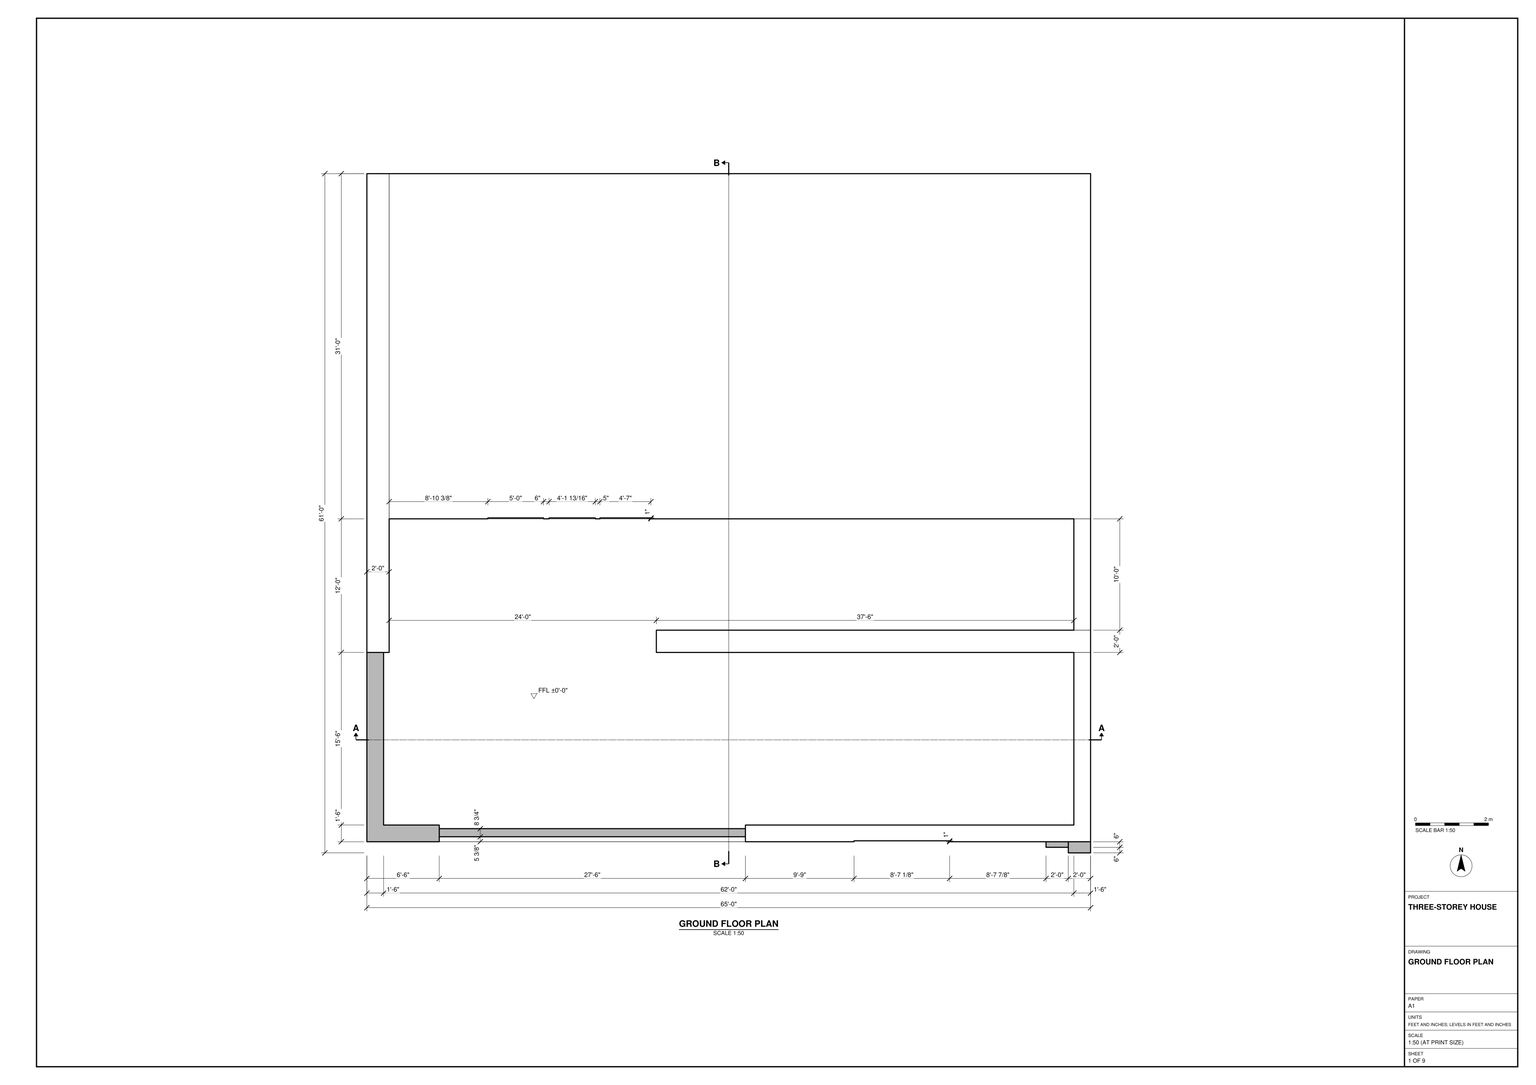
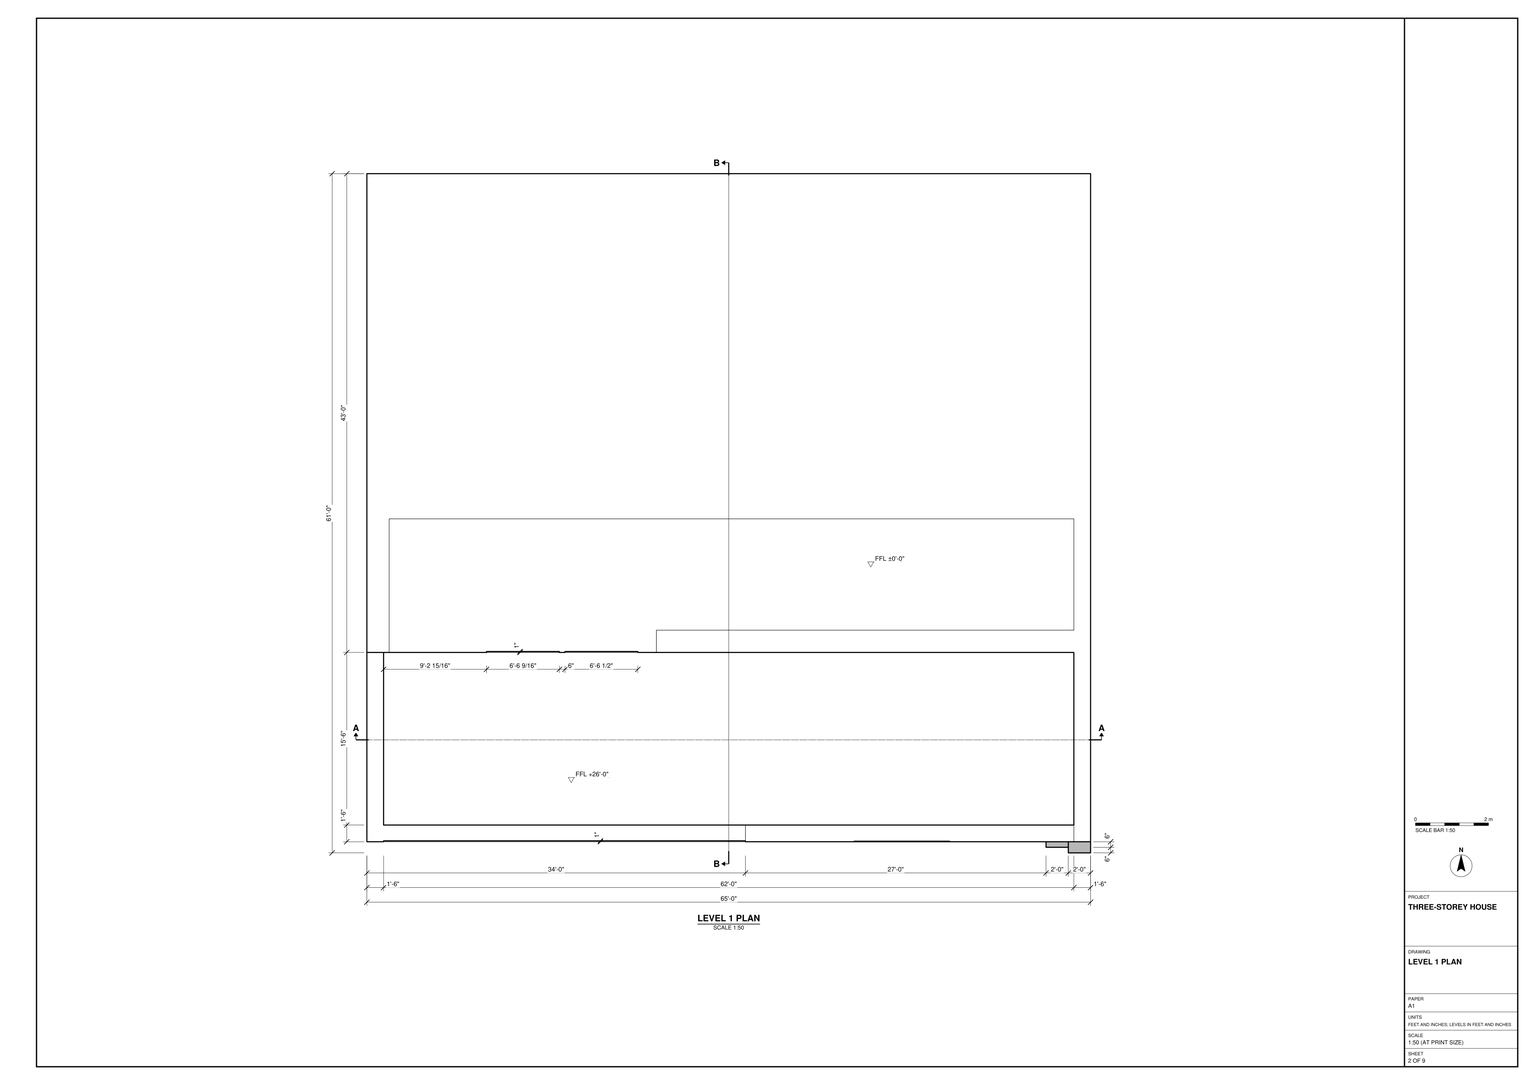
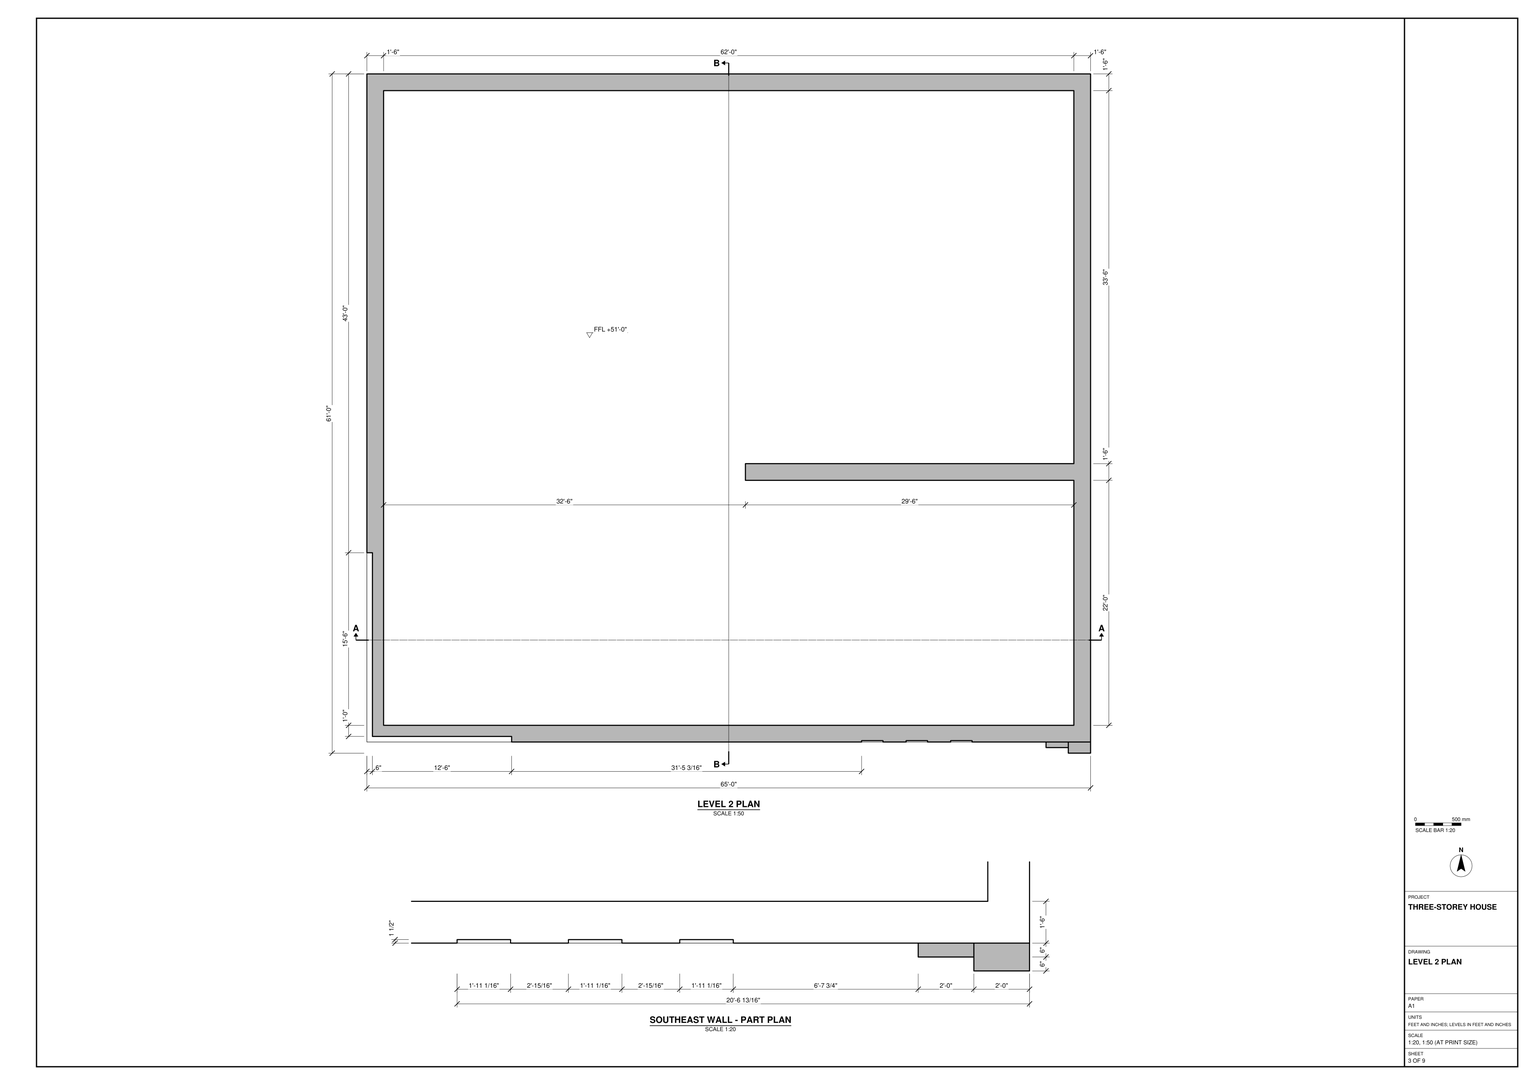
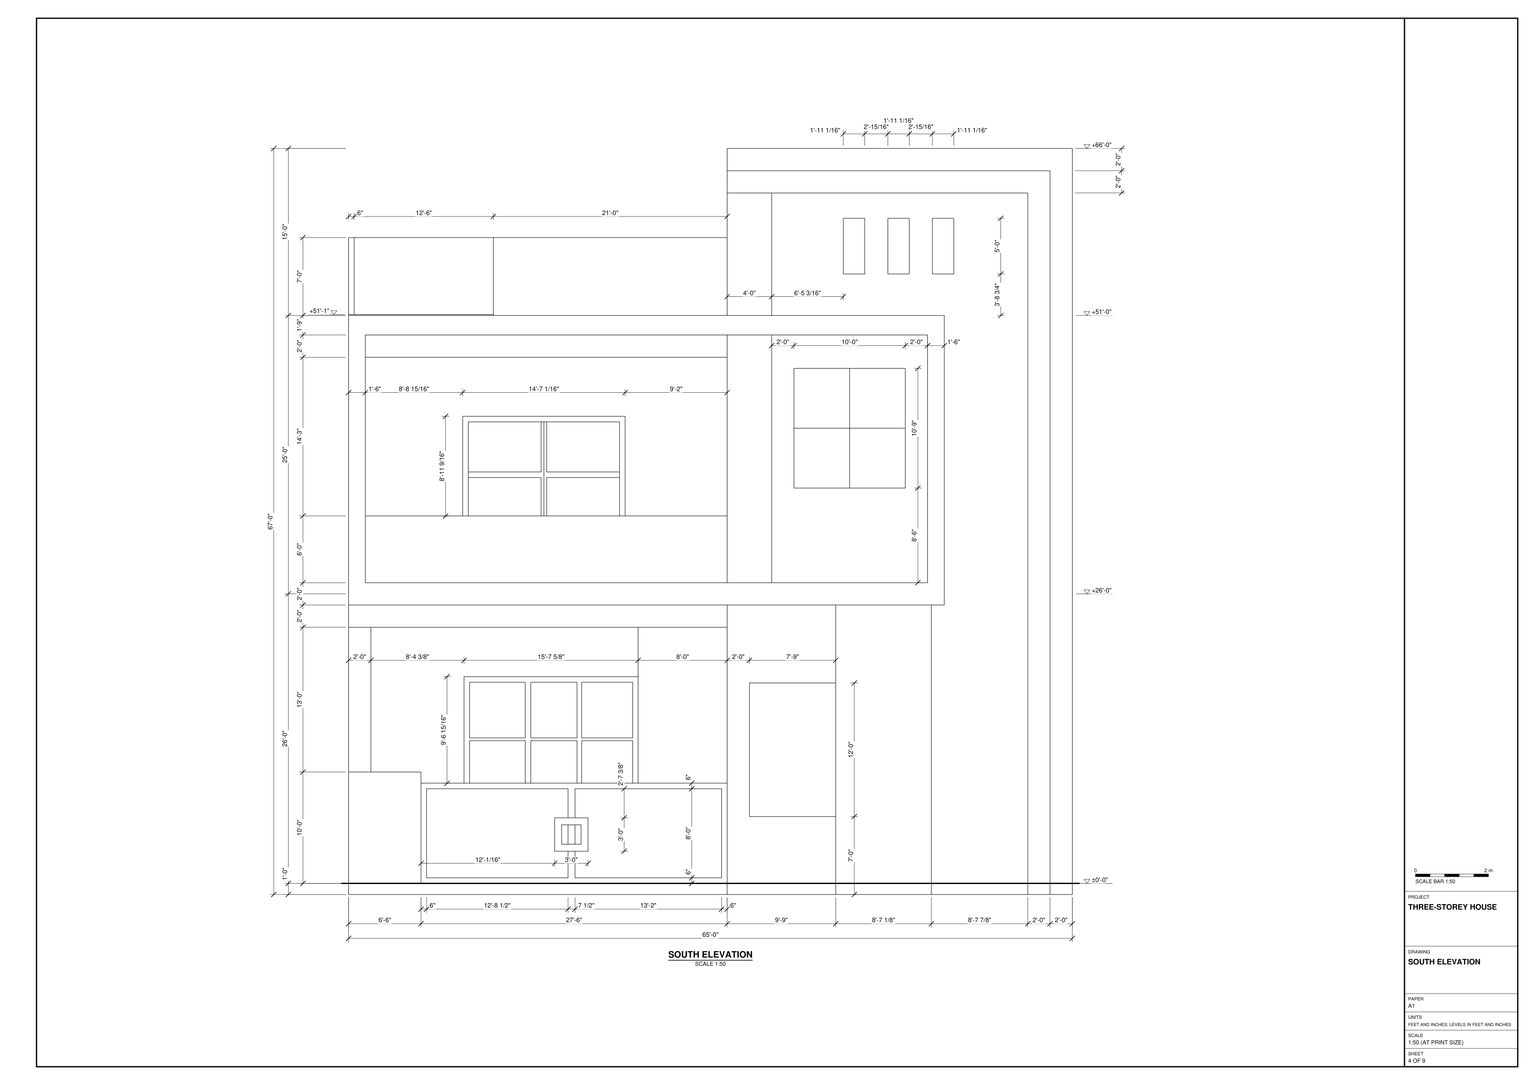
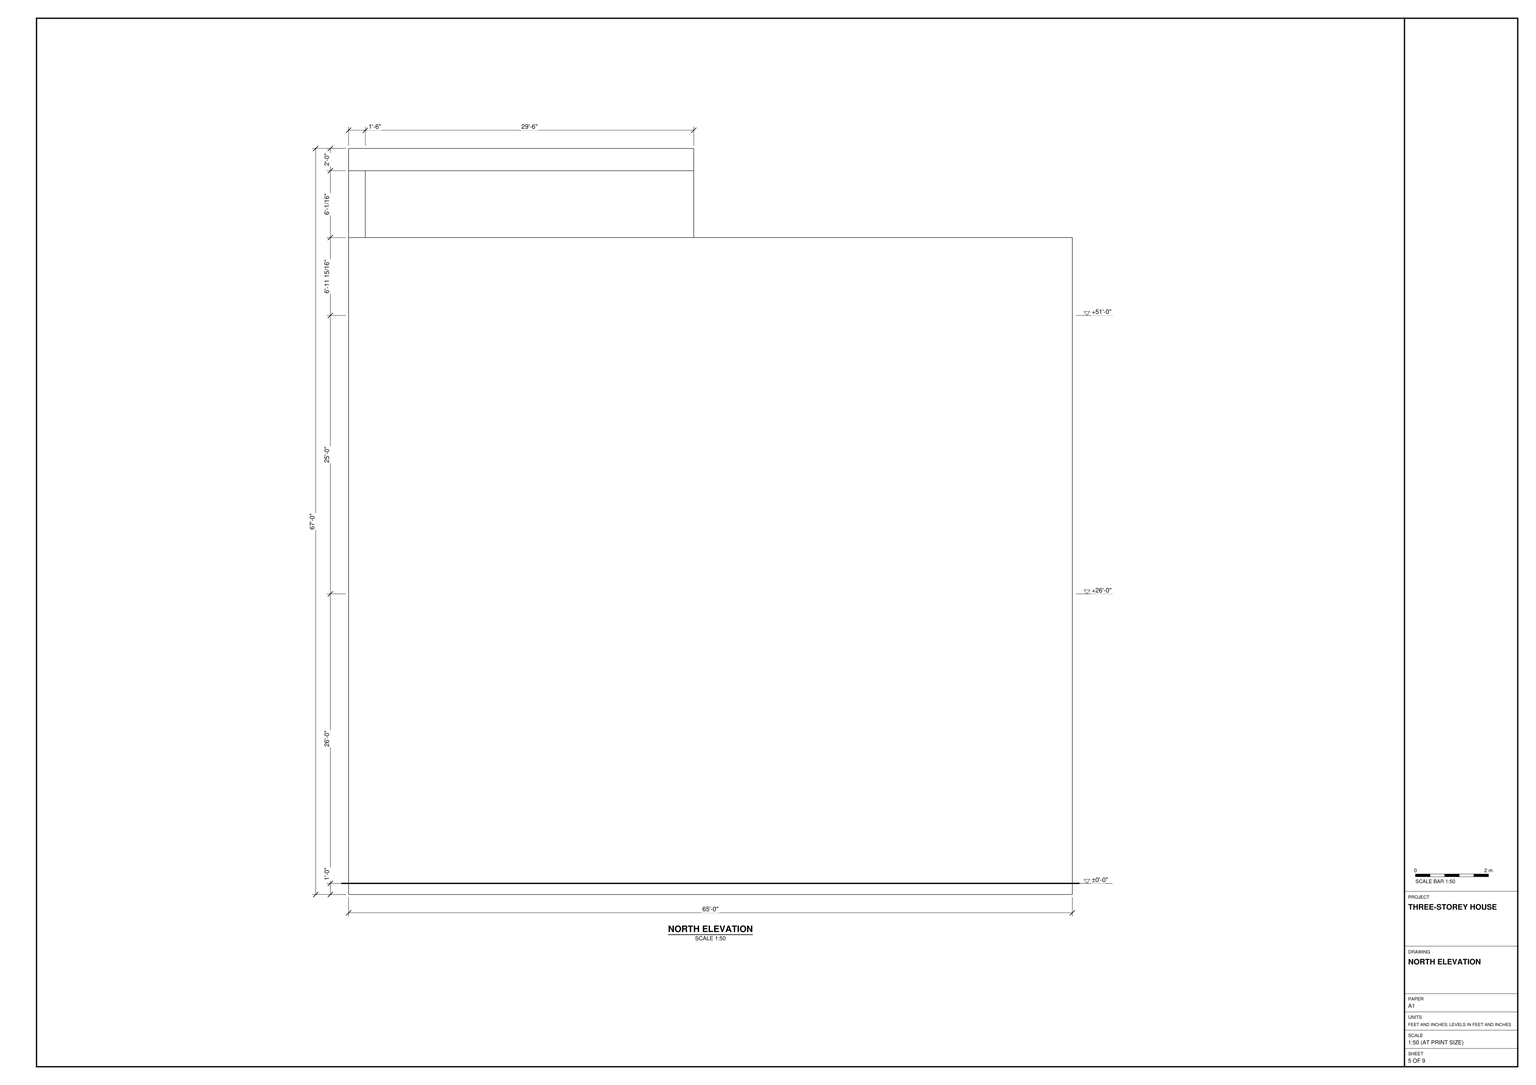
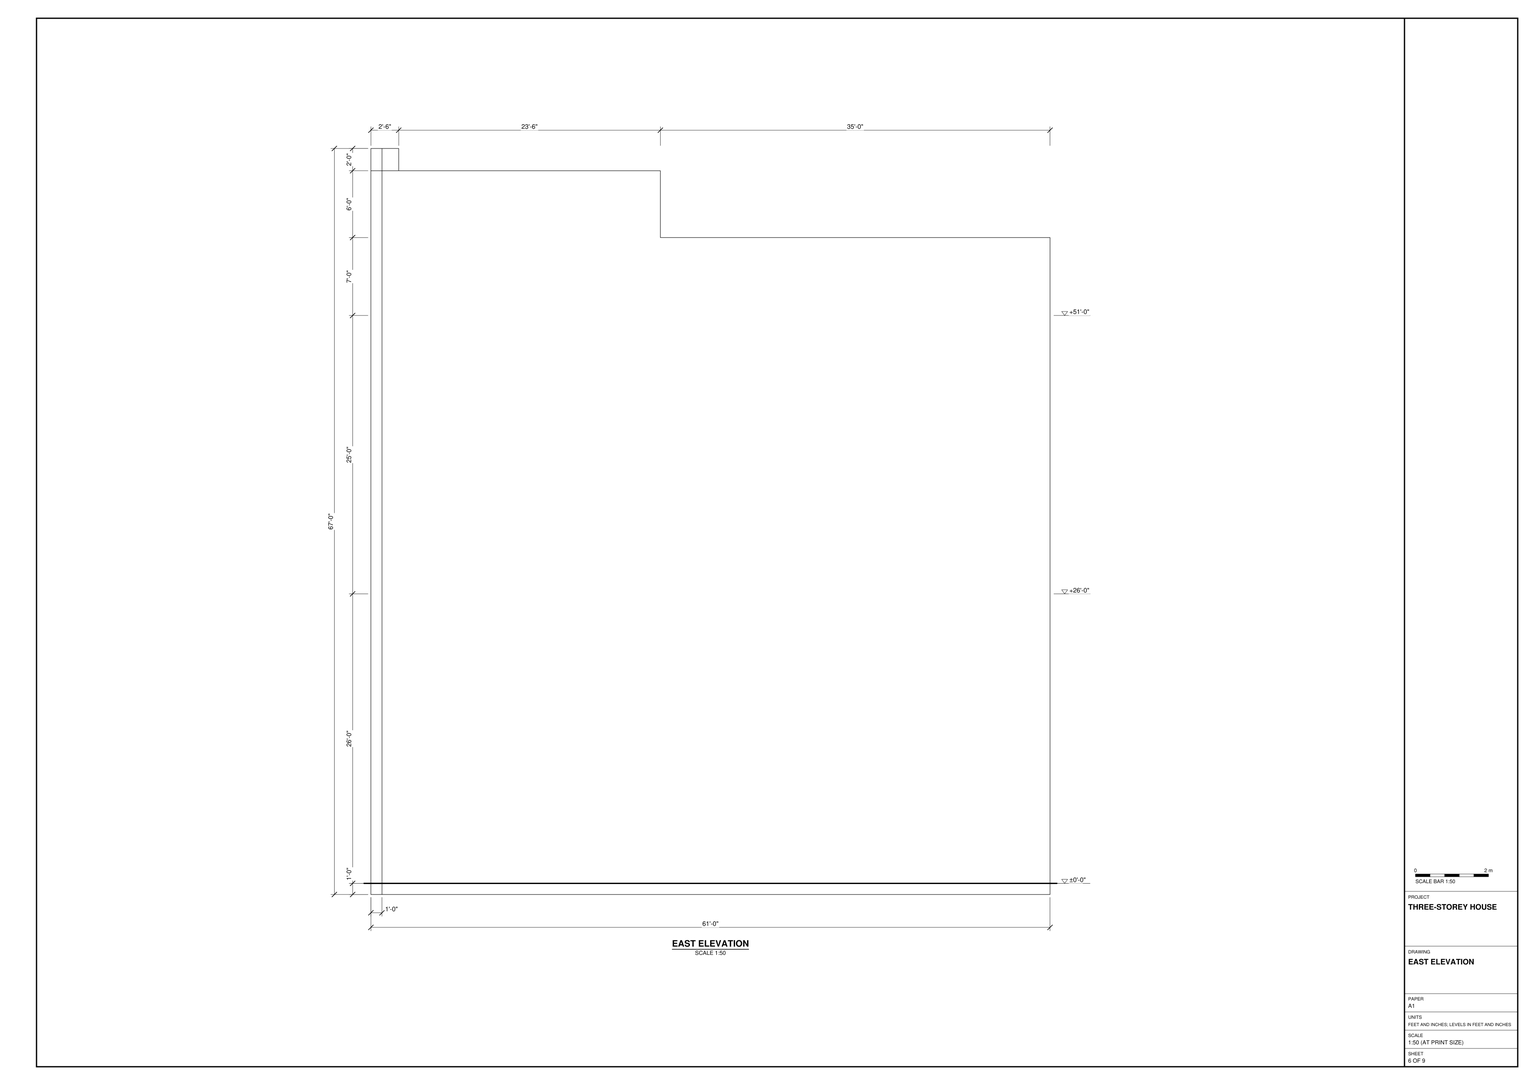
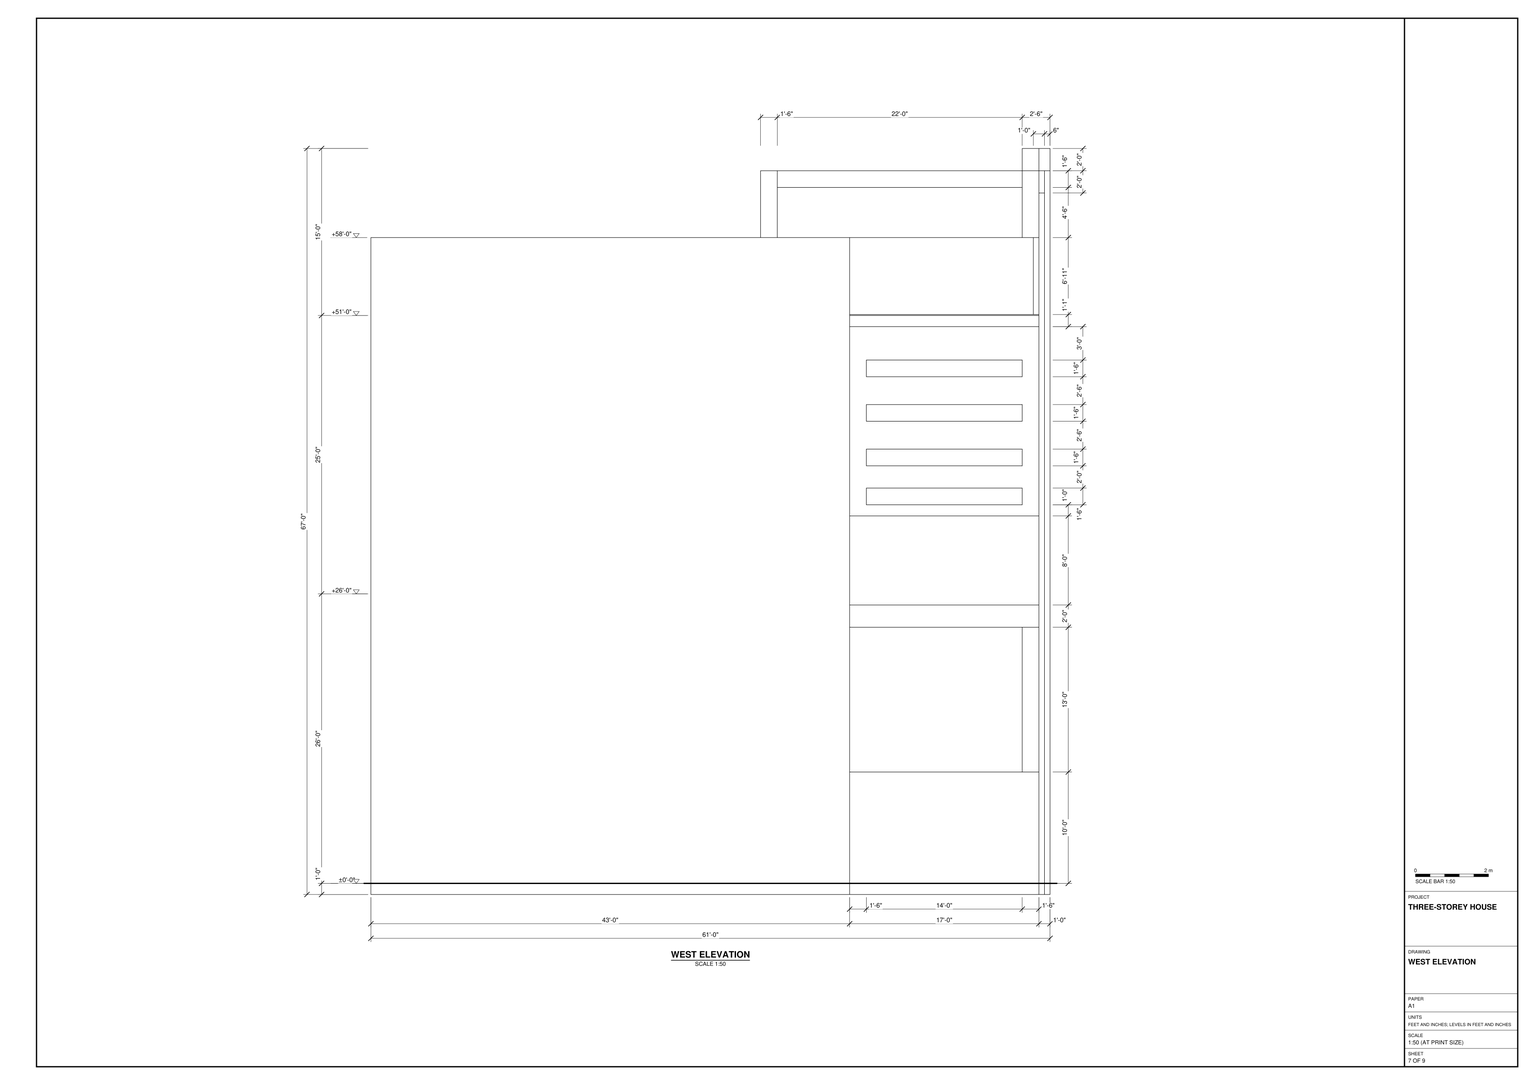
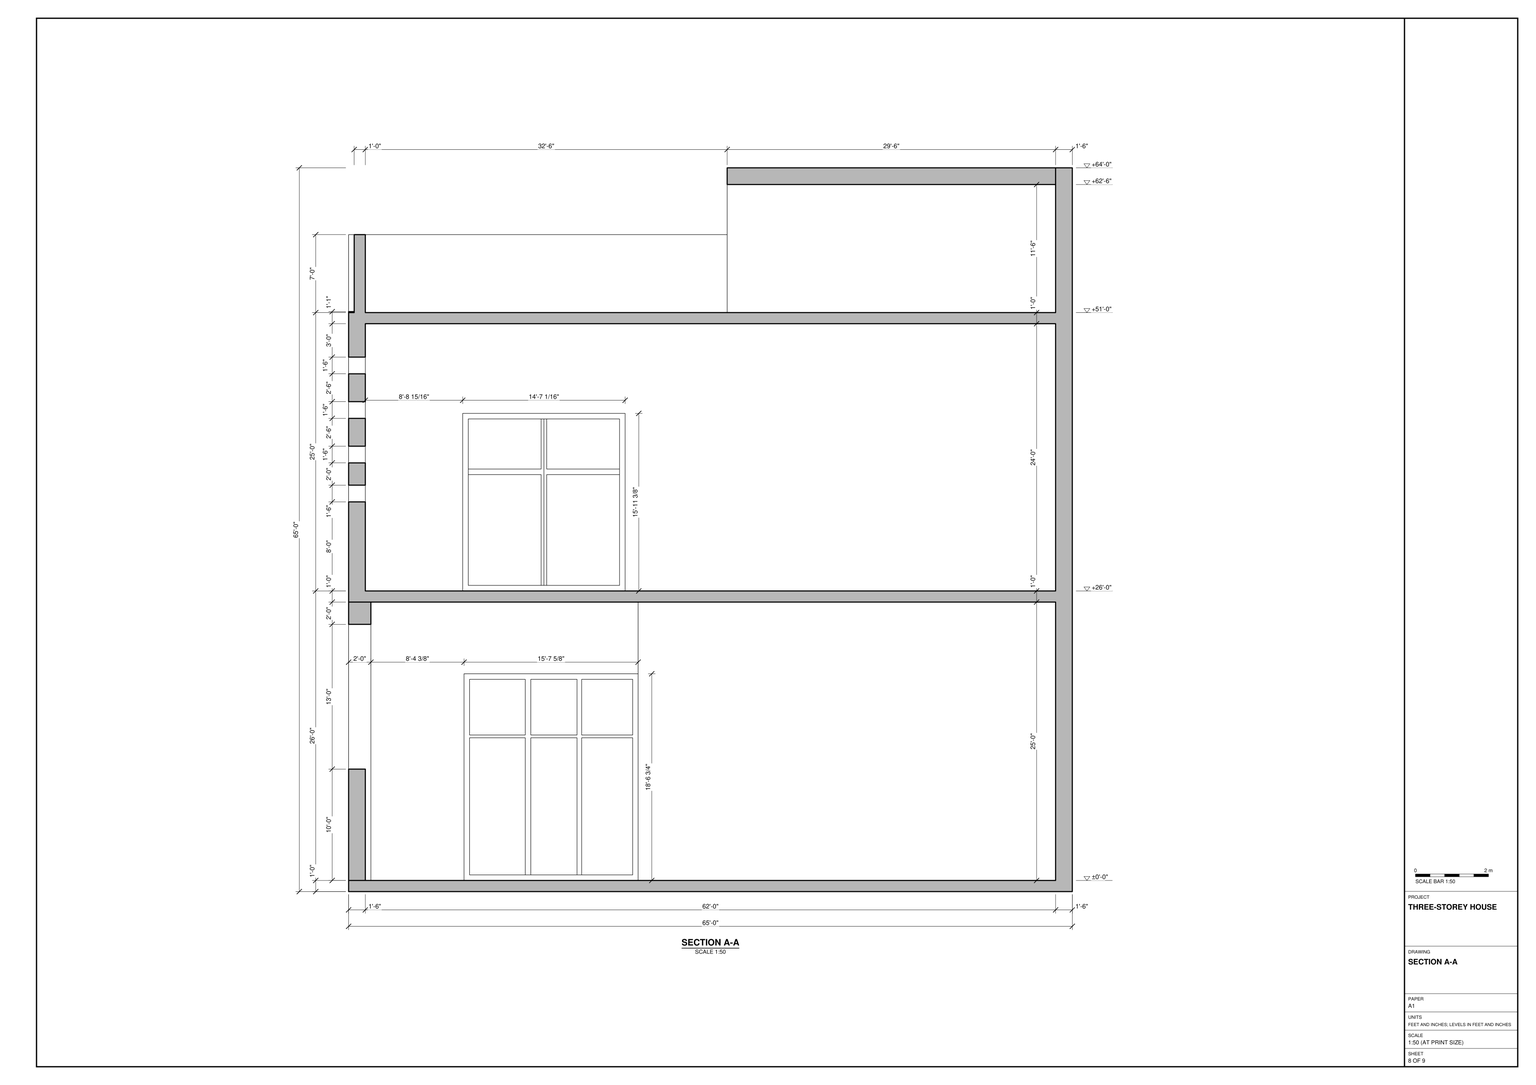
Build the three-storey house in SketchUp using task_files/diagram_01.pdf. Work in feet and inches. Set out the model with its east–west width of 65'-0" along X, its north–south depth of 61'-0" along Y and its overall height of 67'-0" along Z. Use finished floor levels of ±0'-0", +26'-0" and +51'-0".

Use a common north edge to align the plans. Follow the stepped outline on the ground floor and the shallower band along the south side on Level 1 rather than copying one floor outline to the next. On Level 2, model the perimeter walls and the partial wall extending west from the east wall. Use the enlarged southeast wall plan to resolve the shallow changes in the face of the south wall and the steps at its corner.

Build the walls at their drawn thicknesses and use the sections and elevations to locate the slabs, roof, openings and facade projections. Include stairs, built-in joinery and main furniture only where shown. Keep walls, slabs, roof elements and each furniture or joinery piece in separate groups or components, and use components for repeated parts. Any decor or loose items shown may be represented by suitable library components. Save one SketchUp model as output_files/three_storey_house_with_its_stepped_south_facade.skp.

# SketchUp Ruby script. Lengths in inches.
U = 1.inch
M = Sketchup.active_model
def pt(a) = Geom::Point3d.new(a.map { |v| v * U })
def face(e, loops, mat)
  f = e.add_face(loops[0].map { |a| pt(a) })
  loops[1..].each { |l| e.add_face(l.map { |a| pt(a) }).erase! }
  f.material = f.back_material = mat if mat
  f
end
# faces: each face lists its corners as indices into pts; further lists are holes
def faces(e, pts, list, mat = nil) = list.each { |f| face(e, (f[0].is_a?(Array) ? f : [f]).map { |l| l.map { |i| pts[i] } }, mat) }
# xy, xz, yz: faces in a plane at the given z, y or x. An outline is a flat list of corners, or four numbers for a rectangle; further outlines are holes
def ring(l) = l.size == 4 ? [[l[0], l[1]], [l[2], l[1]], [l[2], l[3]], [l[0], l[3]]] : l.each_slice(2).to_a
def flat(e, list, mat, &to3) = list.each { |f| face(e, (f[0].is_a?(Array) ? f : [f]).map { |l| ring(l).map { |u, v| to3.(u, v) } }, mat) }
def xy(e, z, list, mat = nil) = flat(e, list, mat) { |x, y| [x, y, z] }
def xz(e, y, list, mat = nil) = flat(e, list, mat) { |x, z| [x, y, z] }
def yz(e, x, list, mat = nil) = flat(e, list, mat) { |y, z| [x, y, z] }
def lines(e, pts, list) = list.each { |a, b| e.add_line(pt(pts[a]), pt(pts[b])) }
# prism: a flat outline (further loops are holes) pulled along v
def prism(e, loops, v, mat = nil)
  f = face(e, loops, mat); d = Geom::Vector3d.new(v.map { |x| x * U })
  f.pushpull(f.normal.samedirection?(d) ? d.length : -d.length)
end
def box(e, o, s, mat = nil) = prism(e, [[o, [o[0] + s[0], o[1], o[2]], [o[0] + s[0], o[1] + s[1], o[2]], [o[0], o[1] + s[1], o[2]]]], [0, 0, s[2]], mat)
def at(x, y, z, deg = 0) = Geom::Transformation.translation(pt([x, y, z])) * Geom::Transformation.rotation(ORIGIN, Z_AXIS, deg.degrees)
def axes(o, x, y, z) = Geom::Transformation.new([*x, 0, *y, 0, *z, 0, *pt(o).to_a, 1])
def part(name) = M.definitions.add(name)
# library, detail: a bought-in or finely detailed component or shape, given as its bounding box
def library(name, o, s) = part(name).tap { |d| box(d.entities, o, s) }
def detail(e, o, s) = box(e.add_group.entities, o, s)
def put(e, d, t, mat = nil) = e.add_instance(d, t).tap { |i| i.material = mat if mat }
def group(e, t, mat = nil) = e.add_group.tap { |g| g.transformation = t; g.material = mat if mat }.entities
root = M.entities
M.materials.add("[0033_NavajoWhite]").color = [216, 188, 147]
M.materials.add("[0038_Orange]").color = [168, 108, 0]
M.materials.add("[0068_LightGreen]").color = [80, 132, 80]
M.materials.add("[0068_LightGreen]1").color = [100, 165, 100]
M.materials.add("[0068_LightGreen]2").color = [106, 175, 106]
M.materials.add("[0078_DarkSlateGray]").color = [27, 45, 45]
M.materials.add("[0078_DarkSlateGray]1").color = [28, 48, 48]
M.materials.add("[0078_DarkSlateGray]2").color = [21, 35, 35]
M.materials.add("[0078_DarkSlateGray]3").color = [24, 40, 40]
M.materials.add("[0078_DarkSlateGray]4").color = [21, 35, 35]
M.materials.add("[0118_Thistle]").color = [216, 191, 216]
M.materials.add("[Cladding Siding Tan]").color = [73, 70, 70]
M.materials.add("[Cladding Siding White]").color = [137, 137, 137]
M.materials.add("[Siding Rusty Metal]").color = [206, 195, 174]
M.materials.add("[Stone Marble]").color = [143, 138, 136]
M.materials.add("[Stone Sandstone Ashlar Light]").color = [191, 162, 127]
M.materials.add("[Translucent Glass Gray]").color = [32, 66, 33]
M.materials["[Translucent Glass Gray]"].alpha = 0.5
M.materials.add("[Translucent Glass Gray]1").color = [128, 128, 128]
M.materials["[Translucent Glass Gray]1"].alpha = 0.5
M.materials.add("[Wood Veneer 01]").color = [120, 70, 37]
xy(root,0,[[756,0,780,12],[732,6,756,12],[0,12,0,732,780,732,780,12,628.11,12,628.11,13,525,13,525,12]])
xy(root,12,[[0,12,0,216,18,216,18,30,78,30,78,12],[78,17.38,408,26.11],[0,216,24,732],[312,216,780,240],[762,240,780,360],
  [24,360,780,732]])
xy(root,12,[[78,12,408,17.38],[78,26.11,408,26.11,408,30,762,30,762,216,312,216,312,240,762,240,762,360,24,360,24,216,18,216,18,30,78,30]],"[Stone Marble]")
xy(root,18,[[130.37,360,190.37,361],[196.37,360,246.19,361],[251.19,360,306.19,361]])
xy(root,120,[[78,17.38,408,26.11]],"[0078_DarkSlateGray]4")
xy(root,132,[[0,12,78,12,78,30,18,30,18,216,0,216]],"[0078_DarkSlateGray]")
xy(root,165.75,[[130.37,360,190.37,361],[196.37,360,246.19,361],[251.19,360,306.19,361]])
xy(root,168.75,[[130.37,360,190.37,361],[196.37,360,246.19,361],[251.19,360,306.19,361]])
xy(root,228.75,[[130.37,360,190.37,361],[196.37,360,246.19,361],[251.19,360,306.19,361]])
xy(root,288,[[0,12,0,216,24,216,24,30,408,30,408,12]],"[0078_DarkSlateGray]")
xy(root,312,[[0,12,408,12,408,30,24,30,24,216,0,216],[525,12,628.11,13]])
xy(root,312,[[24,30,24,360,762,360,762,240,312,240,312,216,762,216,762,30]],"[0118_Thistle]")
xy(root,324,[[18,30,762,216]],"[Stone Marble]")
xy(root,330,[[128.96,216,207.49,217],[213.49,216,292.02,217]])
xy(root,336,[[18,12,408,13]])
xy(root,408,[[18,13,408,30]],"[0068_LightGreen]")
xy(root,420,[[0,30,18,198]])
xy(root,438,[[480,12,540,13],[540,12,600,13],[0,30,18,198]])
xy(root,449.375,[[128.96,216,207.49,217],[213.49,216,292.02,217]])
xy(root,455.375,[[128.96,216,207.49,217],[213.49,216,292.02,217]])
xy(root,462,[[0,30,18,198]])
xy(root,480,[[0,30,18,198]])
xy(root,509.375,[[128.96,216,207.49,217],[213.49,216,292.02,217]])
xy(root,510,[[0,30,18,198]])
xy(root,528,[[0,30,18,198]])
xy(root,558,[[0,30,18,198]])
xy(root,567,[[480,12,540,13],[540,12,600,13]])
xy(root,576,[[0,30,18,198]])
xy(root,579,[[18,16,408,30]],"[0078_DarkSlateGray]")
xy(root,603,[[18,12,408,16],[18,16,408,30]])
xy(root,612,[[18,30,762,216]],"[0118_Thistle]")
xy(root,624,[[0,12,0,216,6,216,6,18,156,18,156,12],[18,30,762,30,762,294,408,294,408,312,762,312,762,714,18,714]])
xy(root,625,[[0,12,156,12,156,18,6,18,6,216,0,216]])
xy(root,668.75,[[533.2,12,556.26,13.5],[581.2,12,604.26,13.5],[629.2,12,652.26,13.5]])
xy(root,708,[[156,12,408,12,408,30,18,30,18,714,762,714,762,312,780,312,780,732,0,732,0,216,6,216,6,18,156,18]])
xy(root,728.75,[[533.2,12,556.26,13.5],[581.2,12,604.26,13.5],[629.2,12,652.26,13.5]])
xy(root,756,[[408,6,732,12]])
xy(root,762,[[408,30,762,294]])
xy(root,780,[[408,6,756,12]])
xy(root,780,[[408,30,762,294],[762,30,780,30,780,312,408,312,408,294,762,294]],"[0068_LightGreen]2")
xy(root,780,[[408,0,756,6]],"[0078_DarkSlateGray]")
xy(root,804,[[408,0,780,12],[408,12,780,30]],"[0078_DarkSlateGray]1")
xz(root,0,[[756,0,780,0,780,804,408,804,408,780,756,780]],"[0078_DarkSlateGray]")
xz(root,6,[[732,0,756,0,756,780,408,780,408,756,732,756]])
xz(root,12,[[732,0,732,756,408,756,408,780,756,780,756,0],[756,0,756,780,408,780,408,804,780,804,780,0],[[0,312,642,624],[18,336,624,603]],[0,624,156,625]])
xz(root,12,[[[628.11,0,732,0,732,756,456,756,456,624,642,624,642,312,628.11,312],[629.2,668.75,652.26,728.75],[581.2,668.75,604.26,728.75],[533.2,668.75,556.26,728.75]]],"[0068_LightGreen]")
xz(root,12,[[408,0,525,0,525,84,432,84,432,228,525,228,525,312,408,312]],"[0068_LightGreen]1")
xz(root,12,[[0,12,78,132],[0,288,408,312],[156,624,408,708]],"[0078_DarkSlateGray]")
xz(root,12,[[408,336,456,603],[408,624,456,756]],"[Cladding Siding Tan]")
xz(root,12,[[432,84,525,228]],"[Cladding Siding White]")
xz(root,12,[[0,0,408,12]],"[Stone Marble]")
xz(root,12,[[[456,336,624,603],[480,438,600,567]]],"[Stone Sandstone Ashlar Light]")
xz(root,13,[[18,336,408,408]],"[0068_LightGreen]")
xz(root,13,[[525,0,628.11,312]],"[0078_DarkSlateGray]")
xz(root,13,[[480,438,540,502.5],[540,438,600,502.5],[480,502.5,540,567],[540,502.5,600,567]],"[Translucent Glass Gray]")
xz(root,13.5,[[533.2,668.75,556.26,728.75],[581.2,668.75,604.26,728.75],[629.2,668.75,652.26,728.75]],"[0078_DarkSlateGray]")
xz(root,16,[[18,579,408,603]],"[0078_DarkSlateGray]")
xz(root,17.38,[[229.6,54.17,236.5,75.09],[236.5,54.17,244,75.09],[244,54.17,250.52,75.09]])
xz(root,17.38,[[[222.0625,46.63,258.0625,82.63],[229.6,54.17,250.52,75.09]]],"[0038_Orange]")
xz(root,17.38,[[[78,12,408,120],[84,18,84,114,236.5,114,236.5,82.63,244,82.63,244,114,402,114,402,18,244,18,244,46.63,236.5,46.63,236.5,18]]],"[0078_DarkSlateGray]3")
xz(root,17.38,[[84,18,236.5,18,236.5,46.63,222.0625,46.63,222.0625,82.63,236.5,82.63,236.5,114,84,114],[244,18,402,18,402,114,244,114,244,82.63,258.0625,82.63,258.0625,46.63,244,46.63]],"[Siding Rusty Metal]")
xz(root,18,[[6,624,156,625]])
xz(root,18,[[6,625,156,708]],"[Cladding Siding Tan]")
xz(root,26.11,[[78,12,408,120]],"[Siding Rusty Metal]")
xz(root,30,[[0,420,18,438],[0,462,18,480],[0,510,18,528],[0,558,18,576],[18,603,408,612],
  [408,762,762,780]])
xz(root,30,[[408,12,762,312],[408,324,762,612]],"[0033_NavajoWhite]")
xz(root,30,[[18,324,408,408]],"[0068_LightGreen]")
xz(root,30,[[18,12,78,132],[24,288,408,312],[18,579,408,603]],"[0078_DarkSlateGray]")
xz(root,30,[[408,780,780,804]],"[0078_DarkSlateGray]4")
xz(root,30,[[18,624,18,708,408,708,408,762,762,762,762,624]],"[0118_Thistle]")
xz(root,198,[[0,420,18,438],[0,462,18,480],[0,510,18,528],[0,558,18,576]])
xz(root,216,[[0,12,18,108],[0,108,18,132],[0,288,24,312],[0,324,18,408],[0,408,18,612],
  [0,624,6,625],[0,625,6,708]])
xz(root,216,[[18,12,24,12,24,288,0,288,0,132,18,132],[312,12,762,312],[18,324,122.96,324,122.96,515.375,298.02,515.375,298.02,324,762,324,762,612,18,612]],"[0033_NavajoWhite]")
xz(root,216,[[[122.96,324,298.02,515.375],[128.96,330,292.02,509.375]],[207.49,330,210.49,330,210.49,509.375,207.49,509.375,207.49,455.375,128.96,455.375,128.96,449.375,207.49,449.375],[210.49,330,213.49,330,213.49,449.375,292.02,449.375,292.02,455.375,213.49,455.375,213.49,509.375,210.49,509.375]],"[Wood Veneer 01]")
xz(root,217,[[128.96,455.375,207.49,509.375],[213.49,455.375,292.02,509.375]],"[Translucent Glass Gray]")
xz(root,217,[[128.96,330,207.49,449.375],[213.49,330,292.02,449.375]],"[Wood Veneer 01]")
xz(root,240,[[312,12,762,312]],"[0033_NavajoWhite]")
xz(root,294,[[408,762,762,780]])
xz(root,294,[[408,624,762,762]],"[0068_LightGreen]2")
xz(root,312,[[408,624,762,780],[762,708,780,780]],"[0068_LightGreen]2")
xz(root,360,[[24,12,124.37,12,124.37,234.75,312.19,234.75,312.19,12,762,12,762,312,24,312]],"[0033_NavajoWhite]")
xz(root,360,[[[124.37,12,312.19,234.75],[130.37,18,130.37,165.75,190.37,165.75,190.37,18,196.37,18,196.37,165.75,246.19,165.75,246.19,18,251.19,18,251.19,165.75,306.19,165.75,306.19,18],[130.37,168.75,190.37,228.75],[251.19,168.75,306.19,228.75],[196.37,168.75,246.19,228.75]]],"[Wood Veneer 01]")
xz(root,361,[[130.37,168.75,190.37,228.75],[196.37,168.75,246.19,228.75],[251.19,168.75,306.19,228.75]],"[Translucent Glass Gray]1")
xz(root,361,[[130.37,18,190.37,165.75],[196.37,18,246.19,165.75],[251.19,18,306.19,165.75]],"[Wood Veneer 01]")
xz(root,714,[[18,624,762,708]],"[0118_Thistle]")
xz(root,732,[[0,0,780,12],[0,12,780,708]],"[0118_Thistle]")
yz(root,0,[[12,312,216,408],[[12,408,216,612],[30,558,198,576],[30,510,198,528],[30,462,198,480],[30,420,198,438]],[12,612,216,624],[12,624,216,625]])
yz(root,0,[[12,0,216,12],[12,12,216,132],[12,288,216,312]],"[0078_DarkSlateGray]")
yz(root,0,[[216,0,732,12],[216,12,732,708]],"[0118_Thistle]")
yz(root,6,[[18,624,216,625]])
yz(root,6,[[18,625,216,708]],"[Cladding Siding Tan]")
yz(root,18,[[[30,324,216,324,216,612,30,612,30,579,16,579,16,603,12,603,12,408,30,408],[30,462,198,480],[30,510,198,528],[30,558,198,576],[30,420,198,438]],[12,336,13,408],[16,579,30,603]])
yz(root,18,[[30,12,216,132]],"[0078_DarkSlateGray]")
yz(root,18,[[30,624,714,708]],"[0118_Thistle]")
yz(root,24,[[216,12,360,312]],"[0033_NavajoWhite]")
yz(root,24,[[30,288,216,312]],"[0078_DarkSlateGray]2")
yz(root,78,[[17.38,12,26.11,120]])
yz(root,78,[[12,12,17.38,12,17.38,120,26.11,120,26.11,12,30,12,30,132,12,132]],"[0078_DarkSlateGray]")
yz(root,128.96,[[216,330,217,449.375],[216,455.375,217,509.375]])
yz(root,130.37,[[360,18,361,165.75],[360,168.75,361,228.75]])
yz(root,156,[[12,624,18,625],[12,625,18,708]])
yz(root,190.37,[[360,18,361,165.75],[360,168.75,361,228.75]])
yz(root,196.37,[[360,18,361,165.75],[360,168.75,361,228.75]])
yz(root,207.49,[[216,330,217,449.375],[216,455.375,217,509.375]])
yz(root,213.49,[[216,330,217,449.375],[216,455.375,217,509.375]])
yz(root,246.19,[[360,18,361,165.75],[360,168.75,361,228.75]])
yz(root,251.19,[[360,18,361,165.75],[360,168.75,361,228.75]])
yz(root,292.02,[[216,330,217,449.375],[216,455.375,217,509.375]])
yz(root,306.19,[[360,18,361,165.75],[360,168.75,361,228.75]])
yz(root,312,[[216,12,240,312]],"[0033_NavajoWhite]")
yz(root,408,[[17.38,12,26.11,120],[12,288,30,312],[12,336,13,408],[16,579,30,603]])
yz(root,408,[[12,12,12,288,30,288,30,12,26.11,12,26.11,120,17.38,120,17.38,12],[12,408,12,603,16,603,16,579,30,579,30,408]],"[0033_NavajoWhite]")
yz(root,408,[[294,624,312,780],[12,708,30,780],[6,756,12,780],[30,762,294,780],[0,780,12,804],
  [12,780,30,804]],"[0068_LightGreen]2")
yz(root,480,[[12,438,13,502.5],[12,502.5,13,567]])
yz(root,525,[[12,0,13,12],[12,12,13,312]])
yz(root,533.2,[[12,668.75,13.5,728.75]])
yz(root,556.26,[[12,668.75,13.5,728.75]])
yz(root,581.2,[[12,668.75,13.5,728.75]])
yz(root,600,[[12,438,13,502.5],[12,502.5,13,567]])
yz(root,604.26,[[12,668.75,13.5,728.75]])
yz(root,628.11,[[12,0,13,312]])
yz(root,629.2,[[12,668.75,13.5,728.75]])
yz(root,652.26,[[12,668.75,13.5,728.75]])
yz(root,732,[[6,0,12,756]])
yz(root,756,[[6,0,12,780]])
yz(root,756,[[0,0,6,780]],"[0078_DarkSlateGray]")
yz(root,762,[[30,762,294,780]])
yz(root,762,[[30,12,216,312],[240,12,360,312],[30,324,216,612]],"[0033_NavajoWhite]")
yz(root,762,[[30,624,294,762],[312,624,714,708]],"[0118_Thistle]")
yz(root,780,[[0,0,12,12]])
yz(root,780,[[0,12,12,780],[0,780,12,804],[12,780,30,804]],"[0078_DarkSlateGray]2")
yz(root,780,[[12,0,732,12],[12,12,732,12,732,708,312,708,312,780,12,780]],"[0118_Thistle]")
p = [[762,12,312],[762,30,312],[408,12,324],[408,30,324],[408,12,624],[408,30,624]]
lines(root,p,[[0,1],[2,3],[4,5]])
